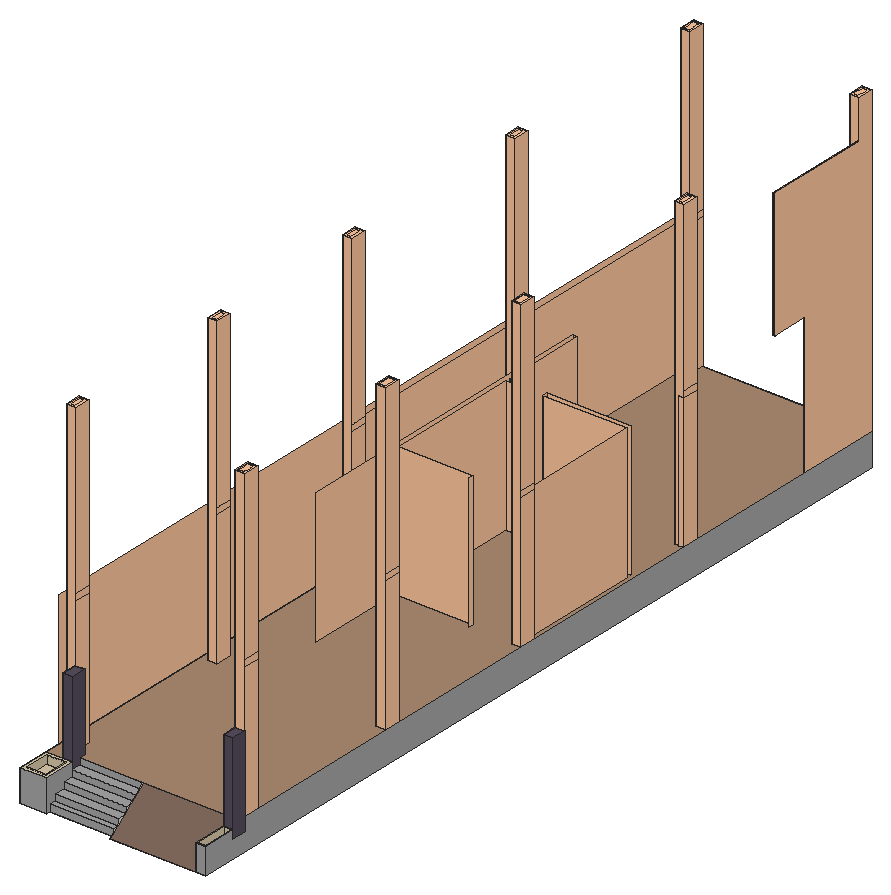
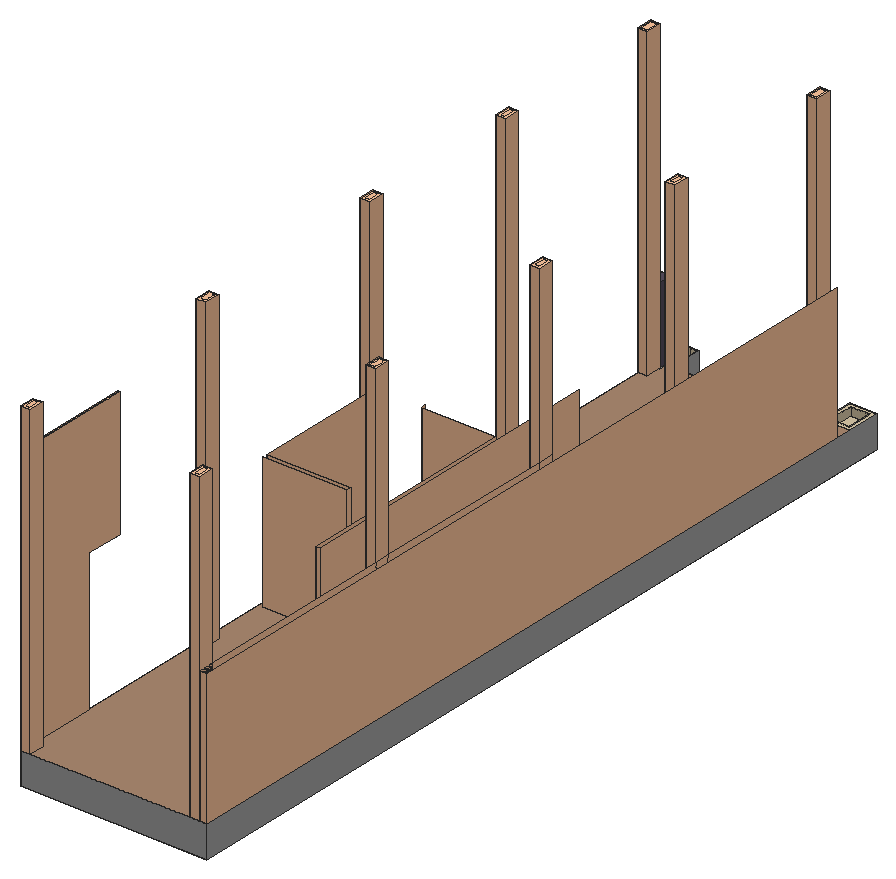
# SketchUp Ruby script. Lengths in inches.
U = 1.inch
M = Sketchup.active_model
def pt(a) = Geom::Point3d.new(a.map { |v| v * U })
def face(e, loops, mat)
  f = e.add_face(loops[0].map { |a| pt(a) })
  loops[1..].each { |l| e.add_face(l.map { |a| pt(a) }).erase! }
  f.material = f.back_material = mat if mat
  f
end
# faces: each face lists its corners as indices into pts; further lists are holes
def faces(e, pts, list, mat = nil) = list.each { |f| face(e, (f[0].is_a?(Array) ? f : [f]).map { |l| l.map { |i| pts[i] } }, mat) }
# xy, xz, yz: faces in a plane at the given z, y or x. An outline is a flat list of corners, or four numbers for a rectangle; further outlines are holes
def ring(l) = l.size == 4 ? [[l[0], l[1]], [l[2], l[1]], [l[2], l[3]], [l[0], l[3]]] : l.each_slice(2).to_a
def flat(e, list, mat, &to3) = list.each { |f| face(e, (f[0].is_a?(Array) ? f : [f]).map { |l| ring(l).map { |u, v| to3.(u, v) } }, mat) }
def xy(e, z, list, mat = nil) = flat(e, list, mat) { |x, y| [x, y, z] }
def xz(e, y, list, mat = nil) = flat(e, list, mat) { |x, z| [x, y, z] }
def yz(e, x, list, mat = nil) = flat(e, list, mat) { |y, z| [x, y, z] }
def lines(e, pts, list) = list.each { |a, b| e.add_line(pt(pts[a]), pt(pts[b])) }
# prism: a flat outline (further loops are holes) pulled along v
def prism(e, loops, v, mat = nil)
  f = face(e, loops, mat); d = Geom::Vector3d.new(v.map { |x| x * U })
  f.pushpull(f.normal.samedirection?(d) ? d.length : -d.length)
end
def box(e, o, s, mat = nil) = prism(e, [[o, [o[0] + s[0], o[1], o[2]], [o[0] + s[0], o[1] + s[1], o[2]], [o[0], o[1] + s[1], o[2]]]], [0, 0, s[2]], mat)
def at(x, y, z, deg = 0) = Geom::Transformation.translation(pt([x, y, z])) * Geom::Transformation.rotation(ORIGIN, Z_AXIS, deg.degrees)
def axes(o, x, y, z) = Geom::Transformation.new([*x, 0, *y, 0, *z, 0, *pt(o).to_a, 1])
def part(name) = M.definitions.add(name)
# library, detail: a bought-in or finely detailed component or shape, given as its bounding box
def library(name, o, s) = part(name).tap { |d| box(d.entities, o, s) }
def detail(e, o, s) = box(e.add_group.entities, o, s)
def put(e, d, t, mat = nil) = e.add_instance(d, t).tap { |i| i.material = mat if mat }
def group(e, t, mat = nil) = e.add_group.tap { |g| g.transformation = t; g.material = mat if mat }.entities
root = M.entities
M.materials.add("[0003_DeepPink]").color = [86, 78, 94]
M.materials.add("[Color A02]1").color = [252, 197, 157]
M.materials.add("[Field Square Tile]").color = [217, 201, 169]
M.materials.add("[Granite Brown]").color = [126, 104, 91]
M.materials.add("[Stone Vein Gray]").color = [166, 165, 165]
M.materials.add("[Tile Veriegated Stone]").color = [171, 137, 112]
c1 = part("Rectangular post")
box(c1.entities,[-0.01,0,-6],[8.99,13.95,85.25],"[0003_DeepPink]")
c2 = part("Rectangular post \#1")
box(c2.entities,[-0.01,0,-6],[8.99,13.95,78],"[0003_DeepPink]")
c3 = part("Rectangular column")
xy(c3.entities,0,[[[0,0.46,8.99,15.39],[2,2,7,13.17]]],"[Color A02]1")
xy(c3.entities,289.125,[[[0,0.46,8.99,15.39],[2,2,7,13.17]],[2,2,7,13.17]],"[Color A02]1")
xz(c3.entities,0.46,[[0,0,8.99,289.125]],"[Color A02]1")
xz(c3.entities,15.39,[[0,0,8.99,289.125]],"[Color A02]1")
yz(c3.entities,0,[[0.46,0,15.39,289.125]],"[Color A02]1")
yz(c3.entities,8.99,[[0.46,0,15.39,125.89],[0.46,125.89,15.39,131.89],[0.46,131.89,15.39,289.125]],"[Color A02]1")
p = [[7,2,0],[7,2,289.125],[2,2,0],[2,2,289.125],[7,13.17,0],[7,13.17,289.125],
  [2,13.17,0],[2,13.17,289.125]]
lines(c3.entities,p,[[0,1],[2,3],[4,5],[6,7]])
c4 = part("Wall section")
xy(c4.entities,0,[[[7.45,-62.8125,7.45,0.46,0,0.46,0,15.39,8.99,15.39,8.99,-62.8125],[2,2,7,13.17]]],"[Color A02]1")
xy(c4.entities,131.89,[[7.45,-98.7,8.98,-62.8125],[8.98,-98.7,8.99,-62.8125]],"[Color A02]1")
xy(c4.entities,251.89,[[7.45,-98.7,8.99,0.46]],"[Color A02]1")
xy(c4.entities,289.125,[[[0,0.46,8.99,15.39],[2,2,7,13.17]],[2,2,7,13.17]],"[Color A02]1")
xz(c4.entities,-98.7,[[7.45,131.89,8.99,251.89]],"[Color A02]1")
xz(c4.entities,-62.8125,[[7.45,0,8.99,131.89]],"[Color A02]1")
xz(c4.entities,0.46,[[0,0,7.45,0,7.45,251.89,8.99,251.89,8.99,289.125,0,289.125]],"[Color A02]1")
xz(c4.entities,15.39,[[0,0,8.99,289.125]],"[Color A02]1")
yz(c4.entities,0,[[0.46,0,15.39,289.125]],"[Color A02]1")
yz(c4.entities,7.45,[[-62.8125,0,-62.8125,131.89,-98.7,131.89,-98.7,251.89,0.46,251.89,0.46,0]],"[Color A02]1")
yz(c4.entities,8.99,[[-62.8125,0,15.39,0,15.39,289.125,0.46,289.125,0.46,251.89,-98.7,251.89,-98.7,131.89,-62.8125,131.89]],"[Color A02]1")
p = [[7,2,0],[7,2,289.125],[2,2,0],[2,2,289.125],[7,13.17,0],[7,13.17,289.125],
  [2,13.17,0],[2,13.17,289.125],[7.46,0.43,251.89],[8.99,0.43,251.89]]
lines(c4.entities,p,[[0,1],[2,3],[4,5],[6,7],[8,9]])
xy(root,-0.11,[[0.89,46.0625,7.86,784.43],[[7.86,371.24,16.85,386.1875],[8.87,372.26,8.87,378.59,9.5,377.95,10.39,377.07,11.28,376.18,12.13,377.04,13.01,376.14,13.89,377.02,13.01,377.92,13.89,378.8,14.77,379.67,15.65,380.55,15.83,380.36,15.83,378.97,15.65,378.78,13.89,377.02,14.77,376.13,15.65,375.23,14.77,374.36,15.65,373.46,15.83,373.27,15.83,372.26,15.2,372.26,14.82,372.64,13.93,373.52,13.05,372.64,12.16,373.52,13.05,374.41,12.16,375.3,11.28,374.41,12.16,373.52,11.28,372.64,10.39,373.52,9.5,372.64,9.12,372.26],[10.375,382.37,9.5,383.27,11.53,385.3,14.57,385.3,14.81,385.03,13.91,384.14,13.04,385.04,13.3,385.3,12.79,385.3,13.04,385.04,12.15,384.14,11.27,385.04,10.38,384.15,9.5,385.04,9.25,385.3,9.76,385.3,9.5,385.04,10.38,384.15,11.26,383.25],[12.13,382.36,11.26,383.25,12.15,384.14,13.02,383.25],[12.13,377.04,11.25,377.93,12.13,378.8125,13.01,377.92],[8.87,380.87,8.87,383.91,9.5,383.27,8.87,382.64,8.87,382.13,9.5,381.49],[15.65,384.11,14.81,385.03,15.07,385.3,15.83,385.3,15.83,384.29],[10.9,372.26,11.28,372.64,11.65,372.26,12.67,372.26,13.05,372.64,13.43,372.26],[15.83,375.04,15.65,375.23,15.83,375.42]],[8.87,372.26,9.12,372.26,9.5,372.64,8.87,373.27],[15.2,372.26,15.83,372.26,15.83,373.27,15.65,373.46,14.82,372.64],[9.5,372.64,10.39,373.52,9.5,374.41,8.87,373.78,8.87,373.27],
  [11.28,372.64,12.16,373.52,11.28,374.41,10.39,373.52],[13.05,372.64,13.93,373.52,13.05,374.41,12.16,373.52],[14.82,372.64,15.65,373.46,14.77,374.36,13.93,373.52],[15.83,373.27,15.83,373.65,15.65,373.46],[15.65,373.46,15.83,373.65,15.83,375.04,15.65,375.23,14.77,374.36],
  [10.39,373.52,11.28,374.41,12.16,375.3,10.39,377.07,9.5,377.95,10.375,378.83,9.5,379.72,8.87,379.09,8.87,380.36,9.5,379.72,10.375,378.83,11.25,379.71,12.13,380.58,11.25,381.48,10.375,380.6,11.25,379.71,10.375,378.83,11.25,377.93,8.87,375.55,8.87,375.04],[13.93,373.52,14.77,374.36,13.89,375.25,13.05,374.41],[8.87,373.78,9.5,374.41,8.87,375.04],[14.77,374.36,15.65,375.23,14.77,376.13,13.89,375.25],[13.05,374.41,13.89,375.25,13.01,376.14,12.16,375.3],
  [15.83,375.04,15.83,375.42,15.65,375.23],[171.33,375.17,171.33,375.42,171.21,375.3],[13.89,375.25,14.77,376.13,13.89,377.02,13.01,376.14],[12.16,375.3,13.01,376.14,12.13,377.04,11.28,376.18],[8.87,375.55,9.5,376.18,8.87,376.82],
  [9.5,376.18,10.39,377.07,9.5,377.95,8.87,377.32,8.87,376.82],[15.83,376.82,15.83,377.19,15.65,377.01],[171.33,376.88,171.33,377.19,171.18,377.04],[15.65,377.01,15.83,377.19,15.83,378.59,15.65,378.78,14.77,377.9],[13.89,377.02,14.77,377.9,13.89,378.8,13.01,377.92],
  [12.13,377.04,13.01,377.92,12.13,378.8125,11.25,377.93],[171.18,377.04,171.33,377.19,171.33,378.65,171.18,378.8125,170.3,377.93],[10.39,377.07,11.25,377.93,10.375,378.83,9.5,377.95],[8.87,377.32,9.5,377.95,8.87,378.59],[14.77,377.9,15.65,378.78,14.77,379.67,13.89,378.8],
  [171.33,378.65,171.33,378.97,171.18,378.8125],[15.65,378.78,15.83,378.97,15.83,380.36,15.65,380.55,14.77,379.67],[12.13,378.8125,13.01,379.69,12.13,380.58,11.25,381.48,10.375,382.37,9.5,381.49,11.25,379.71],[12.13,378.8125,13.01,379.69,12.13,380.58,11.25,379.71],[171.18,378.8125,171.33,378.97,171.33,380.43,171.18,380.58,170.3,379.71],
  [8.87,379.09,9.5,379.72,8.87,380.36],[13.01,379.69,13.89,380.57,13.01,381.46,12.13,380.58],[13.01,379.69,15.65,382.33,14.78,383.23,13.91,384.14,13.02,383.25,13.9,382.35,14.78,383.23,15.65,384.11,15.83,384.29,15.83,385.3,15.07,385.3,14.81,385.03,15.65,384.11,14.78,383.23,13.9,382.35,14.77,381.45,13.9,382.35,12.13,380.58],[171.33,380.43,171.33,380.74,171.18,380.58],[15.65,380.55,15.83,380.74,15.83,382.13,15.65,382.33,15.83,382.51,15.83,382.13,15.65,382.33,14.78,383.23,13.9,382.35,14.77,381.45],
  [15.65,380.55,15.83,380.74,15.83,382.13,15.65,382.33,14.77,381.45],[13.89,380.57,14.77,381.45,13.9,382.35,13.01,381.46],[12.13,380.58,13.01,381.46,12.13,382.36,11.25,381.48],[10.375,380.6,11.25,381.48,10.375,382.37,9.5,381.49],[8.87,380.87,9.5,381.49,8.87,382.13],
  [15.83,382.13,15.83,382.51,15.65,382.33],[13.9,382.35,14.78,383.23,13.91,384.14,13.02,383.25],[12.13,382.36,13.02,383.25,12.15,384.14,11.26,383.25],[10.375,382.37,11.26,383.25,10.38,384.15,9.5,383.27],[8.87,382.64,9.5,383.27,8.87,383.91],
  [15.65,384.11,15.83,384.29,15.83,385.3,15.07,385.3,14.81,385.03],[12.15,384.14,13.04,385.04,12.79,385.3,11.53,385.3,11.27,385.04],[13.91,384.14,14.81,385.03,14.57,385.3,13.3,385.3,13.04,385.04],[9.5,385.04,9.76,385.3,9.25,385.3],[[7.86,563.34,16.85,578.28],[8.87,564.35,8.87,565.36,9.5,564.73,9.12,564.35,9.88,564.35,9.5,564.73,10.39,565.62,9.5,566.5,8.87,567.14,8.87,567.64,9.5,568.28,10.39,567.39,9.5,566.5,10.39,565.62,11.28,566.5,10.39,567.39,11.28,568.28,10.39,569.16,9.5,570.05,10.375,570.92,9.5,571.81,8.87,571.1875,8.87,570.68,9.5,570.05,8.87,569.42,8.87,577.27,14.57,577.27,14.82,577.02,13.92,576.14,14.76,575.3,13.87,574.42,13.03,575.26,13.92,576.14,13.04,577.02,13.3,577.27,12.79,577.27,13.04,577.02,12.14,576.14,11.27,577.02,11.53,577.27,11.02,577.27,11.27,577.02,10.36,576.16,9.45,575.29,10.35,574.4,11.24,573.51,10.34,572.63,9.45,573.52,10.35,574.4,9.45,575.29,8.87,574.73,8.87,574.1,9.45,573.52,8.87,572.96,8.87,572.46,9.5,571.81,11.25,570.03,10.39,569.16,11.28,568.28,12.13,569.13,11.25,570.03,12.1,570.87,12.98,569.99,13.87,570.87,12.98,571.76,13.87,572.65,14.76,571.76,13.87,570.87,12.98,569.99,14.76,568.21,15.64,569.1,15.83,569.29,15.83,567.14,15.64,567.33,14.77,566.45,13.93,565.62,13.05,566.5,12.16,565.62,13.05,564.73,12.67,564.35,13.43,564.35,13.05,564.73,13.93,565.62,14.82,564.73,14.44,564.35],[12.1,570.87,11.21,571.76,12.1,572.65,12.98,571.76]],
  [8.87,564.35,9.12,564.35,9.5,564.73,8.87,565.36],[9.88,564.35,10.9,564.35,11.28,564.73,10.39,565.62,9.5,564.73],[10.9,564.35,11.65,564.35,11.28,564.73,12.16,565.62,11.28,566.5,10.39,565.62,11.28,564.73],[11.65,564.35,12.67,564.35,13.05,564.73,12.16,565.62,11.28,564.73],[13.43,564.35,14.44,564.35,14.82,564.73,13.93,565.62,13.05,564.73],
  [15.2,564.35,15.83,564.35,15.83,565.36,15.65,565.56,14.82,564.73],[15.2,564.35,15.83,564.35,15.83,565.74,14.82,564.73],[9.5,564.73,10.39,565.62,9.5,566.5,8.87,565.87,8.87,565.36],[15.83,565.36,15.83,565.74,15.65,565.56,14.77,566.45,15.64,567.33,14.76,568.21,13.89,567.34,13.01,568.24,12.16,567.39,13.05,566.5,13.89,567.34,15.65,565.56],[12.16,565.62,13.05,566.5,12.16,567.39,11.28,566.5],
  [13.93,565.62,14.77,566.45,13.89,567.34,13.05,566.5],[8.87,565.87,9.5,566.5,8.87,567.14],[173.8125,566.45,174.6875,567.33,173.8,568.21,172.93,567.34],[9.5,566.5,10.39,567.39,9.5,568.28,8.87,567.64,8.87,567.14],[11.28,566.5,12.16,567.39,11.28,568.28,10.39,567.39],
  [15.83,567.14,15.83,567.52,15.64,567.33],[15.64,567.33,15.83,567.52,15.83,568.91,15.64,569.1,14.76,568.21],[13.89,567.34,14.76,568.21,13.87,569.1,13.01,568.24],[172.93,567.34,173.8,568.21,172.92,569.1,172.06,568.24],[12.16,567.39,13.01,568.24,12.13,569.13,11.28,568.28],
  [171.21,567.39,172.06,568.24,171.33,568.97,171.18,569.13,170.32,568.28],[173.8,568.21,174.6875,569.1,173.8,569.99,172.92,569.1],[13.01,568.24,13.87,569.1,12.98,569.99,12.13,569.13],[172.06,568.24,172.92,569.1,172.03,569.99,171.33,569.29,171.33,568.97],[15.83,568.91,15.83,569.29,15.64,569.1],
  [172.92,569.1,173.8,569.99,172.92,570.87,172.03,569.99],[12.13,569.13,12.98,569.99,12.1,570.87,11.25,570.03],[10.39,569.16,11.25,570.03,10.375,570.92,9.5,570.05],[8.87,569.42,9.5,570.05,8.87,570.68],[173.8,569.99,174.6875,570.87,173.8,571.76,172.92,570.87],
  [12.1,570.87,12.98,571.76,12.1,572.65,11.21,571.76],[13.87,570.87,14.76,571.76,13.87,572.65,12.98,571.76],[15.64,570.87,15.83,571.0625,15.83,577.27,15.07,577.27,14.82,577.02,15.64,576.19,15.83,576.38,15.83,576,15.64,576.19,14.76,575.3,13.87,574.42,13.03,575.26,13.92,576.14,15.64,574.42,15.83,574.61,15.83,574.23,15.64,574.42,14.76,573.53,15.64,572.65,15.83,572.84,15.83,572.46,15.64,572.65,14.76,571.76],[15.64,570.87,15.83,571.0625,15.83,572.46,15.64,572.65,14.76,571.76],[172.92,570.87,173.8,571.76,172.92,572.65,172.03,571.76],
  [10.375,570.92,11.21,571.76,10.34,572.63,11.21,571.76,12.1,572.65,11.24,573.51,10.34,572.63,9.5,571.81,8.87,572.46,8.87,571.1875,9.5,571.81],[10.375,570.92,11.21,571.76,10.34,572.63,9.5,571.81],[8.87,571.1875,9.5,571.81,8.87,572.46],[11.21,571.76,12.1,572.65,11.24,573.51,10.34,572.63],[10.34,572.63,11.24,573.51,10.35,574.4,9.45,573.52],
  [12.1,572.65,12.98,573.53,12.13,574.38,11.24,573.51],[12.1,572.65,13.87,574.42,13.03,575.26,12.13,574.38,11.24,573.51],[13.87,572.65,14.76,573.53,13.03,575.26,12.14,576.14,11.25,575.27,12.13,574.38,12.98,573.53],[13.87,572.65,14.76,573.53,13.87,574.42,12.98,573.53],[15.64,572.65,15.83,572.84,15.83,574.23,15.64,574.42,14.76,573.53],
  [8.87,572.96,9.45,573.52,8.87,574.1],[12.13,574.38,13.03,575.26,12.14,576.14,11.25,575.27],[15.64,574.42,15.83,574.61,15.83,576,15.64,576.19,14.76,575.3],[8.87,574.73,9.45,575.29,8.87,575.875],[9.45,575.29,10.36,576.16,9.48,577.03,9.76,577.27,9.25,577.27,9.48,577.03,8.87,576.51,8.87,575.875],
  [12.14,576.14,13.04,577.02,12.79,577.27,11.53,577.27,11.27,577.02],[13.92,576.14,14.82,577.02,14.57,577.27,13.3,577.27,13.04,577.02],[10.36,576.16,11.27,577.02,11.02,577.27,9.76,577.27,9.48,577.03],[15.64,576.19,15.83,576.38,15.83,577.27,15.07,577.27,14.82,577.02],[8.87,576.51,9.48,577.03,9.25,577.27,8.87,577.27],
  [[7.86,769.36,16.85,784.43],[8.87,771.89,8.87,778.48,11.28,776.07,12.16,775.1875,13.05,776.07,13.93,775.1875,13.05,774.3,11.28,772.53,10.39,773.41,9.5,772.53],[15.71,776.96,14.82,777.85,15.71,778.73,15.83,778.61,15.83,778.86,15.71,778.73,13.93,780.51,14.78,781.35,15.65,782.22,14.81,783.15,14.57,783.42,15.07,783.42,14.81,783.15,15.65,782.22,15.83,782.02,15.83,777.09],[11.27,770.76,10.39,771.64,11.28,772.53,12.15,771.66],[15.65,775.25,14.82,776.07,15.71,776.96,15.83,776.83,15.83,775.44],[8.87,780.76,8.87,782.02,9.5,781.39],[14.44,770.375,14.8,770.77,15.2,770.375],[12.67,770.375,13.04,770.76,13.43,770.375],[10.9,770.375,11.27,770.76,11.65,770.375],[9.12,770.375,9.5,770.75,9.88,770.375],[15.83,771.51,15.65,771.7,15.83,771.89]],[8.87,770.375,9.12,770.375,9.5,770.75,10.39,771.64,11.27,770.76,12.15,771.66,13.04,770.76,12.67,770.375,11.65,770.375,11.27,770.76,10.9,770.375,15.2,770.375,14.8,770.77,14.44,770.375,13.43,770.375,13.04,770.76,13.91,771.67,14.8,770.77,15.65,771.7,14.78,772.57,15.65,773.47,15.83,773.29,15.83,775.44,15.65,775.25,15.83,775.06,15.83,773.67,15.65,773.47,14.77,774.35,15.65,775.25,14.82,776.07,15.71,776.96,14.82,777.85,13.93,776.96,13.05,777.85,12.16,778.73,13.05,779.62,12.16,780.51,11.28,779.62,10.39,780.51,9.5,779.62,8.87,780.25,8.87,778.99,10.39,780.51,11.28,781.39,12.16,782.28,13.04,783.16,12.79,783.42,11.53,783.42,11.28,783.16,10.39,782.28,9.5,783.16,9.76,783.42,9.25,783.42,9.5,783.16,10.39,782.28,9.5,781.39,10.39,780.51,11.28,779.62,12.16,778.73,13.05,777.85,12.16,776.96,11.28,776.07,12.16,775.1875,11.28,774.3,10.39,775.1875,11.28,776.07,12.16,776.96,13.05,776.07,13.93,776.96,14.82,776.07,13.93,775.1875,14.77,774.35,15.65,773.47,13.91,771.67,13.04,770.76,12.15,771.66,11.28,772.53,9.5,770.75,8.87,771.39],[8.87,770.375,9.12,770.375,9.5,770.75,8.87,771.39],[9.12,770.375,9.88,770.375,9.5,770.75],[10.9,770.375,11.65,770.375,11.27,770.76],
  [12.67,770.375,13.43,770.375,13.04,770.76],[14.44,770.375,15.2,770.375,14.8,770.77],[11.27,770.76,12.15,771.66,11.28,772.53,10.39,771.64],[14.8,770.77,15.65,771.7,14.78,772.57,13.91,771.67],[15.83,771.51,15.83,771.89,15.65,771.7],
  [8.87,771.89,9.5,772.53,8.87,773.16],[9.5,772.53,10.39,773.41,9.5,774.3,8.87,773.67,8.87,773.16],[11.28,772.53,12.16,773.41,11.28,774.3,10.39,773.41],[15.83,773.29,15.83,773.67,15.65,773.47],[10.39,773.41,11.28,774.3,10.39,775.1875,9.5,776.07,10.39,776.96,9.5,777.85,8.87,777.21,8.87,776.71,9.5,776.07,8.87,775.44,8.87,774.93],
  [12.16,773.41,13.05,774.3,12.16,775.1875,11.28,774.3],[8.87,773.67,9.5,774.3,8.87,774.93],[11.28,774.3,12.16,775.1875,11.28,776.07,10.39,775.1875],[13.05,774.3,13.93,775.1875,13.05,776.07,12.16,775.1875],[14.77,774.35,15.65,775.25,14.82,776.07,13.93,775.1875],
  [15.83,775.06,15.83,775.44,15.65,775.25],[10.39,775.1875,11.28,776.07,10.39,776.96,9.5,776.07],[15.65,775.25,15.83,775.44,15.83,776.83,15.71,776.96,14.82,776.07],[8.87,775.44,9.5,776.07,8.87,776.71],[13.05,776.07,13.93,776.96,13.05,777.85,12.16,776.96],
  [14.82,776.07,15.71,776.96,14.82,777.85,13.93,776.96],[10.39,776.96,11.28,777.85,10.39,778.73,9.5,777.85],[10.39,776.96,11.28,777.85,10.39,778.73,9.5,777.85],[15.71,776.96,15.83,777.09,15.83,782.02,15.65,782.22,14.81,783.15,15.07,783.42,14.57,783.42,14.81,783.15,15.65,782.22,14.78,781.35,13.93,780.51,15.71,778.73,15.83,778.86,15.83,778.61,15.71,778.73,14.82,777.85],[15.71,776.96,15.83,777.09,15.83,778.61,15.71,778.73,14.82,777.85],
  [8.87,777.21,9.5,777.85,8.87,778.48],[11.28,777.85,12.16,778.73,13.05,777.85,14.82,779.62,13.05,781.39,12.16,780.51,13.05,779.62,13.93,780.51,14.78,781.35,15.65,780.45,15.83,780.63,15.83,780.25,15.65,780.45,13.93,778.73,13.05,779.62,11.28,777.85,10.39,778.73,11.28,779.62,12.16,780.51,11.28,781.39,10.39,780.51,11.28,779.62,10.39,778.73],[13.05,777.85,13.93,778.73,13.05,779.62,12.16,778.73],[12.16,778.73,13.05,779.62,12.16,780.51,11.28,779.62],[15.71,778.73,15.83,778.86,15.83,780.25,15.65,780.45,14.82,779.62],
  [8.87,778.99,9.5,779.62,8.87,780.25],[11.28,779.62,12.16,780.51,11.28,781.39,10.39,780.51],[13.05,779.62,13.93,780.51,13.05,781.39,12.16,780.51],[14.82,779.62,15.65,780.45,14.78,781.35,13.93,780.51],[15.65,780.45,15.83,780.63,15.83,782.02,15.65,782.22,14.78,781.35],
  [10.39,780.51,11.28,781.39,10.39,782.28,9.5,781.39],[8.87,780.76,9.5,781.39,8.87,782.02],[11.28,781.39,12.16,782.28,11.28,783.16,10.39,782.28],[12.16,782.28,13.04,783.16,12.79,783.42,11.53,783.42,11.28,783.16],[14.81,783.15,15.07,783.42,14.57,783.42],
  [9.5,783.16,9.76,783.42,9.25,783.42]],"[Color A02]1")
xz(root,375.68,[[57.37,-0.11,126.89,125.89]],"[Color A02]1")
xz(root,501.8,[[57.37,-0.11,63.32,125.89],[92.32,-0.11,171.33,125.89]],"[Color A02]1")
xz(root,506.23,[[57.37,-0.11,63.32,125.89],[92.32,-0.11,171.33,125.89]],"[Color A02]1")
xz(root,563.34,[[171.33,-0.11,175.89,125.89]],"[Color A02]1")
xz(root,585.88,[[52.81,-0.11,57.37,125.89]],"[Color A02]1")
xz(root,784.43,[[0.89,-0.11,7.86,125.89]],"[Color A02]1")
yz(root,0.89,[[46.0625,-0.11,784.43,125.89]],"[Color A02]1")
yz(root,7.86,[[371.24,-0.11,386.1875,125.89],[386.1875,-0.11,563.34,125.89],[563.34,-0.11,578.28,125.89],[578.28,-0.11,769.36,125.89],[769.36,-0.11,784.43,125.89]],"[Color A02]1")
yz(root,52.81,[[283.24,-0.11,585.88,125.89]],"[Color A02]1")
yz(root,57.37,[[375.68,-0.11,501.8,125.89],[506.23,-0.11,585.88,125.89]],"[Color A02]1")
yz(root,63.32,[[501.8,-0.11,506.23,125.89]],"[Color A02]1")
yz(root,92.32,[[501.8,-0.11,506.23,125.89]],"[Color A02]1")
yz(root,126.89,[[371.24,-0.11,375.68,125.89]],"[Color A02]1")
yz(root,171.33,[[386.1875,-0.11,501.8,125.89]],"[Color A02]1")
g1 = group(root,at(0.91,46.0625,-6))
xy(g1,-24,[[0,-46.0625,0,738.37,175,738.37,175,-46.0625,84.9375,-46.0625,84.9375,-42.1875,24.9375,-42.1875,24.9375,-46.0625]])
xy(g1,-18,[[24.9375,-42.1875,84.9375,-36.0625]],"[Stone Vein Gray]")
xy(g1,-17.375,[[166.8,-45.26,174.2,-14.76]],"[Field Square Tile]")
xy(g1,-12,[[24.9375,-36.0625,84.9375,-26.0625]],"[Stone Vein Gray]")
xy(g1,-7.25,[[165.99,-13.95,175,0.05]])
xy(g1,-6,[[24.9375,-26.0625,84.9375,-16.33]],"[Stone Vein Gray]")
xy(g1,-1.875,[[3.35,-42.71,21.58,-18.47]],"[Field Square Tile]")
xy(g1,0,[[15.95,-15.11,24.9375,-0.84]],"[Field Square Tile]")
xy(g1,0,[[24.9375,-16.33,84.9375,-7.14]],"[Stone Vein Gray]")
xy(g1,0.75,[[[165.99,-46.0625,175,-13.95],[166.8,-45.26,174.2,-14.76]]],"[Field Square Tile]")
xy(g1,6,[[[0,-46.0625,24.9375,-15.11],[3.35,-42.71,21.58,-18.47]]],"[Field Square Tile]")
xy(g1,6,[[0,-15.11,15.95,-15.11,15.95,-0.84,24.9375,-0.84,24.9375,-7.14,165.99,-7.14,165.99,0,175,0,175,738.37,0,738.37]],"[Tile Veriegated Stone]")
xz(g1,-46.0625,[[0,-24,24.9375,6],[165.99,-24,175,0.75]],"[Stone Vein Gray]")
xz(g1,-45.26,[[166.8,-17.375,174.2,0.75]],"[Field Square Tile]")
xz(g1,-42.71,[[3.35,-1.875,21.58,6]],"[Field Square Tile]")
xz(g1,-42.1875,[[24.9375,-24,84.9375,-18]],"[Stone Vein Gray]")
xz(g1,-36.0625,[[24.9375,-18,84.9375,-12]],"[Stone Vein Gray]")
xz(g1,-26.0625,[[24.9375,-12,84.9375,-6]],"[Stone Vein Gray]")
xz(g1,-18.47,[[3.35,-1.875,21.58,6]],"[Field Square Tile]")
xz(g1,-16.33,[[24.9375,-6,84.9375,0]],"[Stone Vein Gray]")
xz(g1,-15.11,[[15.95,0,24.9375,6]],"[Field Square Tile]")
xz(g1,-14.76,[[166.8,-17.375,174.2,0.75]],"[Field Square Tile]")
xz(g1,-13.95,[[165.99,-7.25,175,0.75]])
xz(g1,-7.14,[[24.9375,0,84.9375,6]],"[Stone Vein Gray]")
xz(g1,-0.84,[[15.95,0,24.9375,6]],"[Field Square Tile]")
xz(g1,0,[[165.99,5.89,175,6]])
xz(g1,0.05,[[165.99,-7.25,175,0.75]])
xz(g1,738.37,[[0,-24,175,6]],"[Stone Vein Gray]")
yz(g1,0,[[-46.0625,-24,738.37,6]],"[Stone Vein Gray]")
yz(g1,3.35,[[-42.71,-1.875,-18.47,6]],"[Field Square Tile]")
yz(g1,15.95,[[-15.11,0,-14.28,6],[-14.28,0,-0.84,6],[-0.84,0,-0.56,6]],"[Field Square Tile]")
yz(g1,21.58,[[-42.71,-1.875,-18.47,6]],"[Field Square Tile]")
yz(g1,24.9375,[[-7.14,0,-0.84,6]],"[Field Square Tile]")
yz(g1,24.9375,[[-46.0625,-24,-42.1875,-24,-42.1875,-18,-36.0625,-18,-36.0625,-12,-26.0625,-12,-26.0625,-6,-16.33,-6,-16.33,0,-15.11,0,-15.11,6,-46.0625,6]],"[Stone Vein Gray]")
yz(g1,84.9375,[[-46.0625,-24,-42.1875,-21.01,-38.28,-18,-36.0625,-16.29,-30.49,-12,-26.0625,-8.59,-22.71,-6,-16.33,-1.08,-14.92,0,-7.14,6,-7.14,0,-16.33,0,-16.33,-6,-26.0625,-6,-26.0625,-12,-36.0625,-12,-36.0625,-18,-42.1875,-18,-42.1875,-24]])
yz(g1,165.99,[[-13.95,-7.25,0.05,-7.25,0.05,0.75,0,5.89,0,6,-7.14,6,-13.95,0.75]])
yz(g1,165.99,[[-46.0625,-24,-46.0625,0.75,-13.95,0.75]],"[Stone Vein Gray]")
yz(g1,166.8,[[-45.26,-17.375,-14.76,0.75]],"[Field Square Tile]")
yz(g1,174.2,[[-45.26,-17.375,-14.76,0.75]],"[Field Square Tile]")
yz(g1,175,[[-46.0625,-24,738.37,-24,738.37,6,0,6,0,5.89,0.05,0.75,0.05,-7.25,-13.95,-7.25,-13.95,0.75,-46.0625,0.75]],"[Stone Vein Gray]")
p = [[84.9375,-46.0625,-24],[165.99,-46.0625,-24],[165.99,-13.95,0.75],[165.99,-7.14,6],[164.99,-7.14,6],[84.9375,-7.14,6],
  [84.9375,-14.92,0],[84.9375,-16.33,-1.08],[84.9375,-22.71,-6],[84.9375,-26.0625,-8.59],[84.9375,-30.49,-12],[84.9375,-36.0625,-16.29],
  [84.9375,-38.28,-18],[84.9375,-42.1875,-21.01],[175,0.05,0.75],[175,0,5.89],[165.99,0,5.89],[165.99,0.05,0.75],
  [15.95,14.93,5.89],[165.99,15.07,5.89],[166.01,-14.23,0.75],[-0.02,-15.11,6],[0,-15.11,6]]
faces(g1,p,[[0,1,2,3,4,5,6,7,8,9,10,11,12,13]],"[Granite Brown]")
faces(g1,p,[[14,15,16,17]])
lines(g1,p,[[18,19],[20,1],[21,22]])
put(g1,c1,at(166.02,-13.95,-1.25))
put(g1,c2,at(15.96,-15.11,6))
g2 = group(root,at(7.86,46.0625,-0.11))
p = [[168.04,0,126],[168.04,0,132]]
lines(g2,p,[[0,1]])
put(g2,c3,at(0.01,165.91,0.11))
put(g2,c3,at(159.04,-0.46,0.11),"[Color A02]1")
put(g2,c3,at(0,-0.46,0))
put(g2,c3,at(0.01,324.73,0.11))
put(g2,c3,at(0.01,516.83,0.11))
put(g2,c3,at(0,722.98,0.13))
put(g2,c4,at(159.05,722.98,0.11))
put(g2,c3,at(159.04,324.73,0.11))
put(g2,c3,at(159.04,516.83,0.11))
put(g2,c3,at(159.04,165.6875,0.11))
